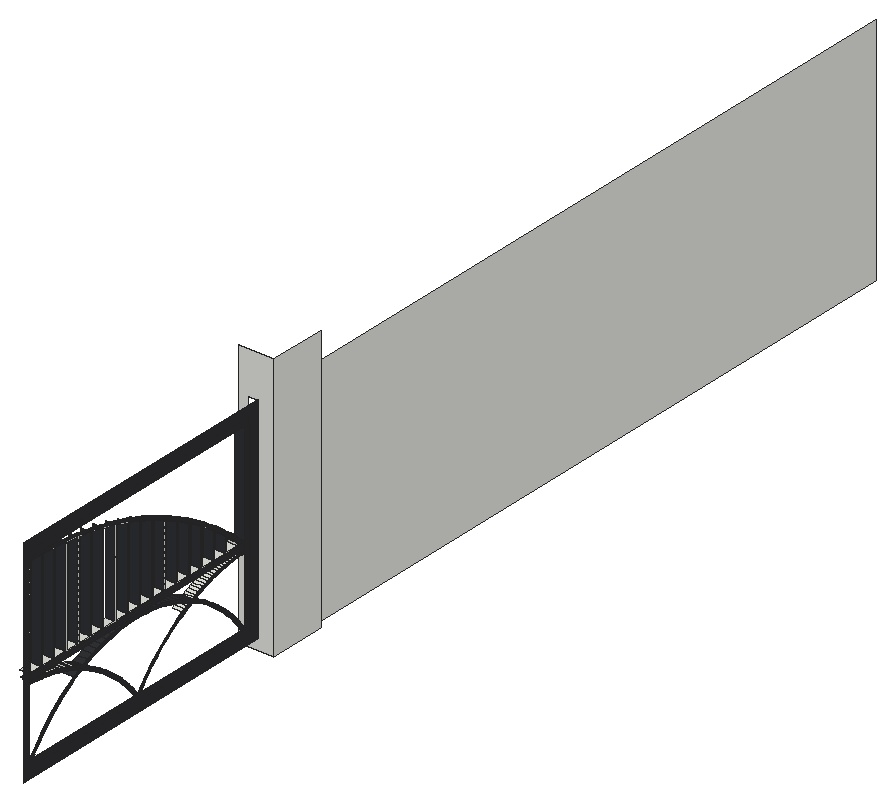
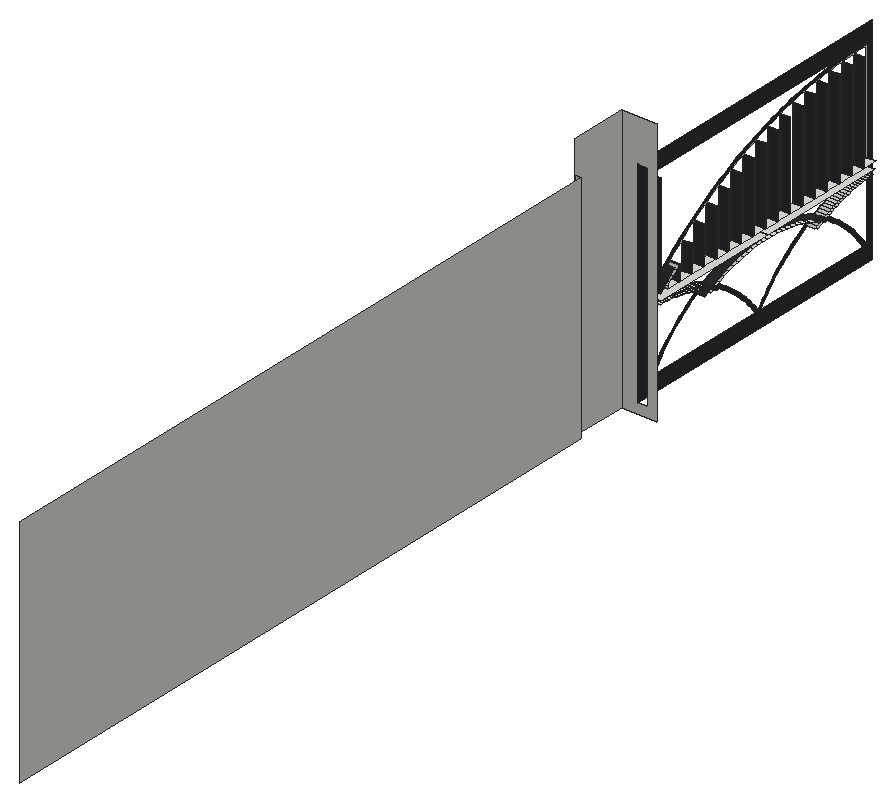
# SketchUp Ruby script. Lengths in inches.
U = 1.inch
M = Sketchup.active_model
def pt(a) = Geom::Point3d.new(a.map { |v| v * U })
def face(e, loops, mat)
  f = e.add_face(loops[0].map { |a| pt(a) })
  loops[1..].each { |l| e.add_face(l.map { |a| pt(a) }).erase! }
  f.material = f.back_material = mat if mat
  f
end
# faces: each face lists its corners as indices into pts; further lists are holes
def faces(e, pts, list, mat = nil) = list.each { |f| face(e, (f[0].is_a?(Array) ? f : [f]).map { |l| l.map { |i| pts[i] } }, mat) }
# xy, xz, yz: faces in a plane at the given z, y or x. An outline is a flat list of corners, or four numbers for a rectangle; further outlines are holes
def ring(l) = l.size == 4 ? [[l[0], l[1]], [l[2], l[1]], [l[2], l[3]], [l[0], l[3]]] : l.each_slice(2).to_a
def flat(e, list, mat, &to3) = list.each { |f| face(e, (f[0].is_a?(Array) ? f : [f]).map { |l| ring(l).map { |u, v| to3.(u, v) } }, mat) }
def xy(e, z, list, mat = nil) = flat(e, list, mat) { |x, y| [x, y, z] }
def xz(e, y, list, mat = nil) = flat(e, list, mat) { |x, z| [x, y, z] }
def yz(e, x, list, mat = nil) = flat(e, list, mat) { |y, z| [x, y, z] }
def lines(e, pts, list) = list.each { |a, b| e.add_line(pt(pts[a]), pt(pts[b])) }
# prism: a flat outline (further loops are holes) pulled along v
def prism(e, loops, v, mat = nil)
  f = face(e, loops, mat); d = Geom::Vector3d.new(v.map { |x| x * U })
  f.pushpull(f.normal.samedirection?(d) ? d.length : -d.length)
end
def box(e, o, s, mat = nil) = prism(e, [[o, [o[0] + s[0], o[1], o[2]], [o[0] + s[0], o[1] + s[1], o[2]], [o[0], o[1] + s[1], o[2]]]], [0, 0, s[2]], mat)
def at(x, y, z, deg = 0) = Geom::Transformation.translation(pt([x, y, z])) * Geom::Transformation.rotation(ORIGIN, Z_AXIS, deg.degrees)
def axes(o, x, y, z) = Geom::Transformation.new([*x, 0, *y, 0, *z, 0, *pt(o).to_a, 1])
def part(name) = M.definitions.add(name)
# library, detail: a bought-in or finely detailed component or shape, given as its bounding box
def library(name, o, s) = part(name).tap { |d| box(d.entities, o, s) }
def detail(e, o, s) = box(e.add_group.entities, o, s)
def put(e, d, t, mat = nil) = e.add_instance(d, t).tap { |i| i.material = mat if mat }
def group(e, t, mat = nil) = e.add_group.tap { |g| g.transformation = t; g.material = mat if mat }.entities
root = M.entities
M.materials.add("ThomThom - Buttons1").color = [48, 49, 53]
xy(root,54,[[474,158.32,477,199.5],[474,199.5,477,241]])
xy(root,56.1,[[474,158.1,477,162.63],[474,162.83,477,167.36],[474,167.56,477,172.09],[474,172.29,477,176.82],[474,177.02,477,181.551],
  [474,181.751,477,186.281],[474,186.481,477,191.011],[474,191.211,477,195.741],[474,195.941,477,200.471],[474,200.671,477,205.201],
  [474,205.401,477,209.931],[474,210.131,477,214.661],[474,214.861,477,219.391],[474,219.591,477,224.122],[474,224.322,477,228.852],
  [474,229.052,477,233.582],[474,233.782,477,238.312]])
xz(root,162.63,[[474,56.1,477,86.87]],"ThomThom - Buttons1")
xz(root,162.83,[[474,56.1,477,86.865]],"ThomThom - Buttons1")
xz(root,167.36,[[474,56.1,477,86.656]],"ThomThom - Buttons1")
xz(root,167.56,[[474,56.1,477,86.642]],"ThomThom - Buttons1")
xz(root,172.09,[[474,56.1,477,86.251]],"ThomThom - Buttons1")
xz(root,172.29,[[474,56.1,477,86.231]],"ThomThom - Buttons1")
xz(root,176.82,[[474,56.1,477,85.652]],"ThomThom - Buttons1")
xz(root,177.02,[[474,56.1,477,85.622]],"ThomThom - Buttons1")
xz(root,181.551,[[474,56.1,477,84.861]],"ThomThom - Buttons1")
xz(root,181.751,[[474,56.1,477,84.822]],"ThomThom - Buttons1")
xz(root,186.281,[[474,56.1,477,83.868]],"ThomThom - Buttons1")
xz(root,186.481,[[474,56.1,477,83.823]],"ThomThom - Buttons1")
xz(root,191.011,[[474,56.1,477,82.67]],"ThomThom - Buttons1")
xz(root,191.211,[[474,56.1,477,82.615]],"ThomThom - Buttons1")
xz(root,195.741,[[474,56.1,477,81.263]],"ThomThom - Buttons1")
xz(root,195.941,[[474,56.1,477,81.198]],"ThomThom - Buttons1")
xz(root,200.471,[[474,56.1,477,79.639]],"ThomThom - Buttons1")
xz(root,200.671,[[474,56.1,477,79.564]],"ThomThom - Buttons1")
xz(root,205.201,[[474,56.1,477,77.781]],"ThomThom - Buttons1")
xz(root,205.401,[[474,56.1,477,77.698]],"ThomThom - Buttons1")
xz(root,209.931,[[474,56.1,477,75.683]],"ThomThom - Buttons1")
xz(root,210.131,[[474,56.1,477,75.59]],"ThomThom - Buttons1")
xz(root,214.661,[[474,56.1,477,73.331]],"ThomThom - Buttons1")
xz(root,214.861,[[474,56.1,477,73.226]],"ThomThom - Buttons1")
xz(root,219.391,[[474,56.1,477,70.706]],"ThomThom - Buttons1")
xz(root,219.591,[[474,56.1,477,70.589]],"ThomThom - Buttons1")
xz(root,224.122,[[474,56.1,477,67.787]],"ThomThom - Buttons1")
xz(root,224.322,[[474,56.1,477,67.658]],"ThomThom - Buttons1")
xz(root,228.852,[[474,56.1,477,64.548]],"ThomThom - Buttons1")
xz(root,229.052,[[474,56.1,477,64.405]],"ThomThom - Buttons1")
xz(root,233.582,[[474,56.1,477,60.952]],"ThomThom - Buttons1")
xz(root,233.782,[[474,56.1,477,60.79]],"ThomThom - Buttons1")
xz(root,238.312,[[474,56.1,477,56.955]])
xz(root,241,[[474,56,477,88]],"ThomThom - Buttons1")
xz(root,246,[[[471,24,482,106],[474,27,477,93]]])
xz(root,264,[[480,24,482,96]])
yz(root,477,[[159.164,32,159.225,32,159.932,33],[199.47,32,199.85,32,199.66,32.254],[239.775,32,239.836,32,239.066,33.003],[[158,56,162.73,56,162.73,86.967,161.629,86.994,160.999,87,158,87],[158.1,56.1,158.1,86.9,160.998,86.9,161.627,86.894,162.63,86.87,162.63,56.1]],[[162.73,56,167.46,56,167.46,86.749,167.048,86.778,165.243,86.878,163.436,86.95,162.73,86.967],[162.83,56.1,162.83,86.865,163.433,86.85,165.238,86.778,167.041,86.679,167.36,86.656,167.36,56.1]],
  [[167.46,56,172.19,56,172.19,86.341,170.652,86.497,168.851,86.651,167.46,86.749],[167.56,56.1,167.56,86.642,168.843,86.552,170.643,86.397,172.09,86.251,172.09,56.1]],[[172.19,56,176.92,56,176.92,85.738,176.038,85.869,174.246,86.105,172.45,86.315,172.19,86.341],[172.29,56.1,172.29,86.231,172.44,86.215,174.234,86.006,176.024,85.77,176.82,85.652,176.82,56.1]],[[176.92,56,181.651,56,181.651,84.944,181.39,84.994,179.611,85.313,177.827,85.604,176.92,85.738],[177.02,56.1,177.02,85.622,177.811,85.506,179.594,85.214,181.372,84.896,181.551,84.861,181.551,56.1]],[[181.651,56,186.381,56,186.381,83.948,184.933,84.276,183.164,84.649,181.651,84.944],[181.751,56.1,181.751,84.822,183.145,84.551,184.912,84.178,186.281,83.868,186.281,56.1]],[[186.381,56,191.111,56,191.111,82.746,190.203,82.996,188.453,83.45,186.696,83.876,186.381,83.948],[186.481,56.1,186.481,83.823,186.674,83.779,188.429,83.353,190.177,82.9,191.011,82.67,191.011,56.1]],
  [[191.111,56,195.841,56,195.841,81.336,195.409,81.477,193.681,82.01,191.946,82.516,191.111,82.746],[191.211,56.1,191.211,82.615,191.919,82.42,193.652,81.914,195.378,81.381,195.741,81.263,195.741,56.1]],[[195.841,56,200.571,56,200.571,79.708,200.539,79.72,198.838,80.332,197.128,80.917,195.841,81.336],[195.941,56.1,195.941,81.198,197.096,80.822,198.805,80.237,200.471,79.639,200.471,56.1]],[[200.571,56,205.301,56,205.301,77.847,203.912,78.42,202.231,79.083,200.571,79.708],[200.671,56.1,200.671,79.564,202.195,78.99,203.875,78.327,205.201,77.781,205.201,56.1]],[[205.301,56,210.031,56,210.031,75.747,208.894,76.277,207.245,77.017,205.584,77.731,205.301,77.847],[205.401,56.1,205.401,77.698,205.545,77.639,207.204,76.925,208.853,76.186,209.931,75.683,209.931,56.1]],[[210.031,56,214.761,56,214.761,73.391,213.773,73.909,212.159,74.723,210.532,75.513,210.031,75.747],[210.131,56.1,210.131,75.59,210.489,75.423,212.114,74.634,213.727,73.82,214.661,73.331,214.661,56.1]],
  [[214.761,56,219.491,56,219.491,70.763,218.537,71.32,216.962,72.207,215.374,73.07,214.761,73.391],[214.861,56.1,214.861,73.226,215.327,72.982,216.914,72.12,218.488,71.233,219.391,70.706,219.391,56.1]],[[219.491,56,224.222,56,224.222,67.841,223.179,68.516,221.646,69.474,220.099,70.409,219.491,70.763],[219.591,56.1,219.591,70.589,220.048,70.323,221.594,69.389,223.125,68.431,224.122,67.787,224.122,56.1]],[[224.222,56,228.952,56,228.952,64.599,227.687,65.502,226.2,66.529,224.697,67.534,224.222,67.841],[224.322,56.1,224.322,67.658,224.642,67.45,226.143,66.447,227.629,65.42,228.852,64.548,228.852,56.1]],[[228.952,56,233.682,56,233.682,61,233.474,61.168,232.052,62.285,230.614,63.379,229.158,64.452,228.952,64.599],[229.052,56.1,229.052,64.405,229.1,64.371,230.554,63.299,231.991,62.205,233.412,61.09,233.582,60.952,233.582,56.1]],[[233.682,56,238.412,56,238.412,57,237.635,57.691,236.266,58.871,234.879,60.03,233.682,61],[233.782,56.1,233.782,60.79,234.815,59.953,236.201,58.795,237.569,57.615,238.312,56.955,238.312,56.1]]])
yz(root,477,[[156,27,246,27,246,93,156,93,156,90,243,90,243,30,156,30],[[156,30,243,90],[158,32,241,88]],[158,32,159.164,32,159.932,33,159.934,33.003,161.1,34.524,162.325,35.997,163.606,37.422,164.942,38.796,166.331,40.117,167.769,41.382,169.256,42.591,170.79,43.741,172.366,44.83,173.984,45.856,175.641,46.819,177.334,47.717,178.417,48.238,179.061,48.548,179.578,48.772,180.819,49.31,182.605,50.004,184.417,50.628,186.252,51.18,188.107,51.661,189.979,52.069,191.866,52.403,193.764,52.664,195.671,52.85,197.584,52.962,199.5,53,201.416,52.962,203.329,52.85,205.236,52.664,207.134,52.403,209.021,52.069,210.893,51.661,212.748,51.18,214.583,50.628,216.395,50.004,218.181,49.31,219.589,48.7,219.939,48.548,220.805,48.131,221.666,47.717,223.359,46.819,225.016,45.856,226.634,44.83,228.21,43.741,229.744,42.591,231.231,41.382,232.669,40.117,234.058,38.796,235.394,37.422,236.675,35.997,237.9,34.524,239.066,33.003,239.836,32,241,32,239.871,33.597,238.681,35.148,237.432,36.652,236.124,38.105,234.761,39.507,233.345,40.855,231.876,42.146,230.359,43.379,228.795,44.552,227.186,45.664,225.535,46.711,223.845,47.694,222.117,48.609,222.001,48.665,220.779,49.253,220.355,49.457,218.562,50.236,216.739,50.943,214.89,51.58,213.018,52.143,211.125,52.634,209.215,53.05,207.29,53.391,205.353,53.657,203.407,53.848,201.455,53.962,199.5,54,197.545,53.962,195.593,53.848,193.647,53.657,191.71,53.391,189.785,53.05,187.875,52.634,185.982,52.143,184.11,51.58,182.261,50.943,180.438,50.236,178.645,49.457,178.376,49.328,177.281,48.801,176.883,48.609,175.155,47.694,173.465,46.711,171.814,45.664,170.205,44.552,168.641,43.379,167.124,42.146,165.655,40.855,164.239,39.507,162.876,38.105,161.568,36.652,160.319,35.148,159.129,33.597],[198.633,32,199.47,32,199.66,32.254,199.268,32.779,198.671,33.547,198.061,34.304,197.437,35.05,196.8,35.784,196.149,36.507,195.486,37.218,194.81,37.918,194.122,38.604,193.421,39.279,192.708,39.94,191.984,40.589,191.248,41.225,190.501,41.847,189.742,42.455,188.973,43.05,188.193,43.631,187.403,44.198,186.602,44.751,185.792,45.288,184.973,45.812,184.144,46.32,183.306,46.814,182.459,47.292,181.604,47.755,180.74,48.202,179.869,48.634,179.731,48.7,179.578,48.772,179.061,48.548,178.417,48.238,180.288,47.31,181.136,46.871,181.975,46.417,182.806,45.947,183.629,45.463,184.442,44.964,185.247,44.45,186.042,43.922,186.827,43.38,187.603,42.824,188.368,42.254,189.123,41.67,189.868,41.073,190.601,40.462,191.324,39.838,192.035,39.201,192.734,38.552,193.422,37.89,194.097,37.216,194.761,36.53,195.412,35.832,196.05,35.122,196.675,34.401,197.288,33.669],[199.85,32,200.687,32,201.493,33,202.032,33.669,202.645,34.401,203.27,35.122,203.908,35.832,204.559,36.53,205.222,37.216,205.898,37.89,206.586,38.552,207.285,39.201,207.996,39.838,208.719,40.462,209.452,41.073,210.197,41.67,210.952,42.254,211.717,42.824,212.493,43.38,213.278,43.922,214.073,44.45,214.878,44.964,215.691,45.463,216.514,45.947,217.345,46.417,218.184,46.871,219.032,47.31,219.609,47.597,220.805,48.131,219.939,48.548,219.589,48.7,219.451,48.634,218.58,48.202,217.716,47.755,216.861,47.292,216.014,46.814,215.176,46.32,214.347,45.812,213.528,45.288,212.718,44.751,211.917,44.198,211.127,43.631,210.347,43.05,209.578,42.455,208.819,41.847,208.072,41.225,207.336,40.589,206.612,39.94,205.899,39.279,205.198,38.604,204.51,37.918,203.834,37.218,203.171,36.507,202.52,35.784,201.883,35.05,201.259,34.304,200.649,33.547,200.052,32.779,199.66,32.254],
  [222.001,48.665,223.165,49.186,223.38,49.274,224.269,49.619,225.165,49.948,226.067,50.261,226.974,50.558,227.887,50.838,228.804,51.102,229.726,51.349,230.652,51.58,231.582,51.793,232.516,51.991,233.453,52.171,234.394,52.334,235.337,52.481,236.282,52.61,237.23,52.722,238.18,52.818,239.131,52.896,240,52.951,241,53.015,241,54,240.029,53.955,239.058,53.893,238.089,53.814,237.121,53.716,236.156,53.602,235.192,53.47,234.231,53.321,233.273,53.155,232.318,52.971,231.367,52.77,230.419,52.552,229.475,52.317,228.536,52.065,227.601,51.796,226.672,51.511,225.748,51.209,224.829,50.89,223.916,50.554,223.01,50.203,222.109,49.835,221.216,49.45,220.779,49.253],[177.281,48.801,178.376,49.328,178.104,49.45,177.211,49.835,176.31,50.203,175.404,50.554,174.491,50.89,173.572,51.209,172.648,51.511,171.718,51.796,170.784,52.065,169.845,52.317,168.901,52.552,167.953,52.77,167.002,52.971,166.047,53.155,165.089,53.321,164.128,53.47,163.164,53.602,162.199,53.716,161.231,53.814,160.262,53.893,159.291,53.955,158.32,54,158,54,158,53.014,159.236,52.957,160.189,52.896,161.14,52.818,162.09,52.722,163.038,52.61,163.983,52.481,164.926,52.334,165.867,52.171,166.804,51.991,167.738,51.793,168.668,51.58,169.594,51.349,170.516,51.102,171.433,50.838,172.346,50.558,173.253,50.261,174.155,49.948,175.051,49.619,175.94,49.274],[158,54,241,56],[239.537,56,241,56,239.656,57.232,238.294,58.443,236.913,59.633,235.514,60.802,234.098,61.95,232.664,63.076,231.213,64.18,229.745,65.261,228.262,66.32,226.762,67.356,225.246,68.37,223.715,69.36,222.17,70.326,220.609,71.269,219.035,72.1875,217.446,73.082,215.845,73.953,214.23,74.799,212.602,75.62,210.962,76.416,209.31,77.187,207.647,77.932,205.972,78.653,204.286,79.347,202.59,80.016,200.885,80.659,199.169,81.275,197.444,81.866,195.711,82.43,193.969,82.967,192.219,83.478,190.461,83.962,188.696,84.42,186.925,84.85,185.147,85.253,183.363,85.629,181.574,85.977,179.779,86.299,177.98,86.593,176.177,86.859,174.37,87.098,172.559,87.309,170.745,87.493,168.929,87.648,167.11,87.776,165.29,87.877,163.468,87.949,161.646,87.994,161.003,88,158,88,158,87,160.999,87,161.629,86.994,162.73,86.967,163.436,86.95,165.243,86.878,167.048,86.778,167.46,86.749,168.851,86.651,170.652,86.497,172.19,86.341,172.45,86.315,174.246,86.105,176.038,85.869,176.92,85.738,177.827,85.604,179.611,85.313,181.39,84.994,181.651,84.944,183.164,84.649,184.933,84.276,186.381,83.948,186.696,83.876,188.453,83.45,190.203,82.996,191.111,82.746,191.946,82.516,193.681,82.01,195.409,81.477,195.841,81.336,197.128,80.917,198.838,80.332,200.539,79.72,200.571,79.708,202.231,79.083,203.912,78.42,205.301,77.847,205.584,77.731,207.245,77.017,208.894,76.277,210.031,75.747,210.532,75.513,212.159,74.723,213.773,73.909,214.761,73.391,215.374,73.07,216.962,72.207,218.537,71.32,219.491,70.763,220.099,70.409,221.646,69.474,223.179,68.516,224.222,67.841,224.697,67.534,226.2,66.529,227.687,65.502,228.952,64.599,229.158,64.452,230.614,63.379,232.052,62.285,233.474,61.168,233.682,61,234.879,60.03,236.266,58.871,237.635,57.691,238.412,57],[238.412,56,239.537,56,238.412,57]],"ThomThom - Buttons1")
yz(root,480,[[264,24,480,96]])
yz(root,482,[[246,24,264,106]])
p = [[477,180.288,47.31],[477,178.417,48.238],[474,178.417,48.238],[474,180.288,47.31],[477,216.861,47.292],[477,217.716,47.755],
  [474,217.716,47.755],[474,216.861,47.292],[477,219.609,47.597],[477,219.032,47.31],[474,219.032,47.31],[474,219.609,47.597],
  [477,220.805,48.131],[474,220.805,48.131],[477,175.155,47.694],[477,176.883,48.609],[474,176.883,48.609],[474,175.155,47.694],
  [477,177.334,47.717],[474,177.334,47.717],[477,221.666,47.717],[474,221.666,47.717],[477,222.117,48.609],[477,223.845,47.694],
  [474,223.845,47.694],[474,222.117,48.609],[477,180.74,48.202],[477,181.604,47.755],[474,181.604,47.755],[474,180.74,48.202],
  [477,218.58,48.202],[474,218.58,48.202],[477,179.869,48.634],[474,179.869,48.634],[477,219.451,48.634],[474,219.451,48.634],
  [477,177.281,48.801],[474,177.281,48.801],[477,179.731,48.7],[474,179.731,48.7],[477,219.589,48.7],[474,219.589,48.7],
  [477,222.001,48.665],[474,222.001,48.665],[477,179.578,48.772],[474,179.578,48.772],[477,218.181,49.31],[474,218.181,49.31],
  [477,223.165,49.186],[474,223.165,49.186],[477,175.94,49.274],[474,175.94,49.274],[477,180.819,49.31],[474,180.819,49.31],
  [477,223.38,49.274],[474,223.38,49.274],[477,175.051,49.619],[474,175.051,49.619],[477,178.104,49.45],[477,178.376,49.328],
  [474,178.376,49.328],[474,178.104,49.45],[477,178.645,49.457],[474,178.645,49.457],[477,182.605,50.004],[474,182.605,50.004],
  [477,216.395,50.004],[474,216.395,50.004],[477,220.355,49.457],[477,220.779,49.253],[474,220.779,49.253],[474,220.355,49.457],
  [477,221.216,49.45],[474,221.216,49.45],[477,224.269,49.619],[474,224.269,49.619],[477,177.211,49.835],[474,177.211,49.835],
  [477,180.438,50.236],[474,180.438,50.236],[477,218.562,50.236],[474,218.562,50.236],[477,222.109,49.835],[474,222.109,49.835],
  [477,174.155,49.948],[474,174.155,49.948],[477,225.165,49.948],[474,225.165,49.948],[477,176.31,50.203],[474,176.31,50.203],
  [477,223.01,50.203],[474,223.01,50.203],[477,173.253,50.261],[474,173.253,50.261],[477,226.067,50.261],[474,226.067,50.261],
  [477,184.417,50.628],[474,184.417,50.628],[477,214.583,50.628],[474,214.583,50.628],[477,175.404,50.554],[474,175.404,50.554],
  [477,182.261,50.943],[474,182.261,50.943],[477,216.739,50.943],[474,216.739,50.943],[477,223.916,50.554],[474,223.916,50.554],
  [477,172.346,50.558],[474,172.346,50.558],[477,226.974,50.558],[474,226.974,50.558],[477,171.433,50.838],[474,171.433,50.838],
  [477,174.491,50.89],[474,174.491,50.89],[477,186.252,51.18],[474,186.252,51.18],[477,212.748,51.18],[474,212.748,51.18],
  [477,224.829,50.89],[474,224.829,50.89],[477,227.887,50.838],[474,227.887,50.838],[477,170.516,51.102],[474,170.516,51.102],
  [477,228.804,51.102],[474,228.804,51.102],[477,173.572,51.209],[474,173.572,51.209],[477,184.11,51.58],[474,184.11,51.58],
  [477,214.89,51.58],[474,214.89,51.58],[477,225.748,51.209],[474,225.748,51.209],[477,169.594,51.349],[474,169.594,51.349],
  [477,229.726,51.349],[474,229.726,51.349],[477,172.648,51.511],[474,172.648,51.511],[477,188.107,51.661],[474,188.107,51.661],
  [477,210.893,51.661],[474,210.893,51.661],[477,226.672,51.511],[474,226.672,51.511],[477,168.668,51.58],[474,168.668,51.58],
  [477,230.652,51.58],[474,230.652,51.58],[477,171.718,51.796],[474,171.718,51.796],[477,227.601,51.796],[474,227.601,51.796],
  [477,167.738,51.793],[474,167.738,51.793],[477,185.982,52.143],[474,185.982,52.143],[477,213.018,52.143],[474,213.018,52.143],
  [477,231.582,51.793],[474,231.582,51.793],[477,189.979,52.069],[474,189.979,52.069],[477,209.021,52.069],[474,209.021,52.069],
  [477,166.804,51.991],[474,166.804,51.991],[477,170.784,52.065],[474,170.784,52.065],[477,228.536,52.065],[474,228.536,52.065],
  [477,232.516,51.991],[474,232.516,51.991],[477,165.867,52.171],[474,165.867,52.171],[477,233.453,52.171],[474,233.453,52.171],
  [477,169.845,52.317],[474,169.845,52.317],[477,187.875,52.634],[474,187.875,52.634],[477,191.866,52.403],[474,191.866,52.403],
  [477,207.134,52.403],[474,207.134,52.403],[477,211.125,52.634],[474,211.125,52.634],[477,229.475,52.317],[474,229.475,52.317],
  [477,164.926,52.334],[474,164.926,52.334],[477,234.394,52.334],[474,234.394,52.334],[477,163.983,52.481],[474,163.983,52.481],
  [477,168.901,52.552],[474,168.901,52.552],[477,230.419,52.552],[474,230.419,52.552],[477,235.337,52.481],[474,235.337,52.481],
  [477,193.764,52.664],[474,193.764,52.664],[477,205.236,52.664],[474,205.236,52.664],[477,163.038,52.61],[474,163.038,52.61],
  [477,236.282,52.61],[474,236.282,52.61],[477,162.09,52.722],[474,162.09,52.722],[477,167.953,52.77],[474,167.953,52.77],
  [477,189.785,53.05],[474,189.785,53.05],[477,209.215,53.05],[474,209.215,53.05],[477,231.367,52.77],[474,231.367,52.77],
  [477,237.23,52.722],[474,237.23,52.722],[477,161.14,52.818],[474,161.14,52.818],[477,195.671,52.85],[474,195.671,52.85],
  [477,203.329,52.85],[474,203.329,52.85],[477,238.18,52.818],[474,238.18,52.818],[477,160.189,52.896],[474,160.189,52.896],
  [477,167.002,52.971],[474,167.002,52.971],[477,232.318,52.971],[474,232.318,52.971],[477,239.131,52.896],[474,239.131,52.896],
  [477,159.236,52.957],[474,159.236,52.957],[477,197.584,52.962],[474,197.584,52.962],[477,201.416,52.962],[474,201.416,52.962],
  [477,240,52.951],[474,240,52.951],[477,166.047,53.155],[474,166.047,53.155],[477,191.71,53.391],[474,191.71,53.391],
  [477,199.5,53],[474,199.5,53],[477,207.29,53.391],[474,207.29,53.391],[477,233.273,53.155],[474,233.273,53.155],
  [477,241,53.015],[474,241,53.015],[477,165.089,53.321],[474,165.089,53.321],[477,234.231,53.321],[474,234.231,53.321],
  [477,164.128,53.47],[474,164.128,53.47],[477,235.192,53.47],[474,235.192,53.47],[477,193.647,53.657],[474,193.647,53.657],
  [477,205.353,53.657],[474,205.353,53.657],[477,163.164,53.602],[474,163.164,53.602],[477,236.156,53.602],[474,236.156,53.602],
  [477,162.199,53.716],[474,162.199,53.716],[477,237.121,53.716],[474,237.121,53.716],[477,161.231,53.814],[474,161.231,53.814],
  [477,195.593,53.848],[474,195.593,53.848],[477,203.407,53.848],[474,203.407,53.848],[477,238.089,53.814],[474,238.089,53.814],
  [477,160.262,53.893],[474,160.262,53.893],[477,197.545,53.962],[474,197.545,53.962],[477,201.455,53.962],[474,201.455,53.962],
  [477,239.058,53.893],[474,239.058,53.893],[477,159.291,53.955],[474,159.291,53.955],[477,240.029,53.955],[474,240.029,53.955],
  [477,158.32,54],[474,158.32,54],[477,199.5,54],[474,199.5,54],[477,241,54],[474,241,54],
  [477,239.656,57.232],[477,241,56],[474,241,56],[474,239.656,57.232],[477,238.312,56.955],[477,237.569,57.615],
  [474,237.569,57.615],[474,238.312,56.955],[477,238.294,58.443],[474,238.294,58.443],[477,236.201,58.795],[474,236.201,58.795],
  [477,236.913,59.633],[474,236.913,59.633],[477,234.815,59.953],[474,234.815,59.953],[477,235.514,60.802],[474,235.514,60.802],
  [477,233.782,60.79],[474,233.782,60.79]]
faces(root,p,[[0,1,2,3],[4,5,6,7],[8,9,10,11],[12,8,11,13],[1,18,19,2],[20,12,13,21],[26,27,28,29],[5,30,31,6],
  [32,26,29,33],[30,34,35,31],[38,32,33,39],[34,40,41,35],[44,38,39,45],[40,46,47,41],[48,42,43,49],[36,50,51,37],
  [52,44,45,53],[54,48,49,55],[50,56,57,51],[58,59,60,61],[64,52,53,65],[46,66,67,47],[69,72,73,70],[74,54,55,75],
  [76,58,61,77],[72,82,83,73],[56,84,85,57],[86,74,75,87],[88,76,77,89],[82,90,91,83],[84,92,93,85],[94,86,87,95],
  [96,64,65,97],[66,98,99,67],[100,88,89,101],[90,106,107,91],[92,108,109,93],[110,94,95,111],[108,112,113,109],[114,100,101,115],
  [116,96,97,117],[98,118,119,99],[106,120,121,107],[122,110,111,123],[112,124,125,113],[126,122,123,127],[128,114,115,129],[120,134,135,121],
  [124,136,137,125],[138,126,127,139],[140,128,129,141],[142,116,117,143],[118,144,145,119],[134,146,147,135],[136,148,149,137],[150,138,139,151],
  [152,140,141,153],[146,154,155,147],[148,156,157,149],[162,150,151,163],[164,142,143,165],[144,166,167,145],[156,168,169,157],[170,152,153,171],
  [154,172,173,155],[174,162,163,175],[168,176,177,169],[178,174,175,179],[180,170,171,181],[184,164,165,185],[166,186,187,167],[172,190,191,173],
  [176,192,193,177],[194,178,179,195],[192,196,197,193],[198,180,181,199],[190,200,201,191],[202,194,195,203],[204,184,185,205],[186,206,207,187],
  [196,208,209,197],[210,202,203,211],[208,212,213,209],[214,198,199,215],[200,220,221,201],[222,210,211,223],[212,224,225,213],[226,204,205,227],
  [206,228,229,207],[230,222,223,231],[224,232,233,225],[234,214,215,235],[220,236,237,221],[238,230,231,239],[232,240,241,233],[242,226,227,243],
  [228,244,245,229],[246,238,239,247],[248,234,235,249],[252,242,243,253],[244,252,253,245],[236,256,257,237],[258,246,247,259],[260,248,249,261],
  [256,262,263,257],[264,260,261,265],[262,266,267,263],[272,264,265,273],[266,274,275,267],[276,272,273,277],[274,278,279,275],[280,276,277,281],
  [278,286,287,279],[288,280,281,289],[286,294,295,287],[296,288,289,297],[294,298,299,295],[300,296,297,301],[298,304,305,299],[310,311,312,313],
  [311,316,317,312],[316,320,321,317],[320,324,325,321]])
faces(root,p,[[14,15,16,17],[22,23,24,25],[15,36,37,16],[42,22,25,43],[59,62,63,60],[68,69,70,71],[62,78,79,63],[80,68,71,81],
  [78,102,103,79],[104,80,81,105],[102,130,131,103],[132,104,105,133],[130,158,159,131],[160,132,133,161],[158,182,183,159],[188,160,161,189],
  [182,216,217,183],[218,188,189,219],[216,250,251,217],[254,218,219,255],[250,268,269,251],[270,254,255,271],[268,282,283,269],[284,270,271,285],
  [282,290,291,283],[292,284,285,293],[290,302,303,291],[302,292,293,303],[306,307,308,309],[314,306,309,315],[318,314,315,319],[322,318,319,323]],"ThomThom - Buttons1")
